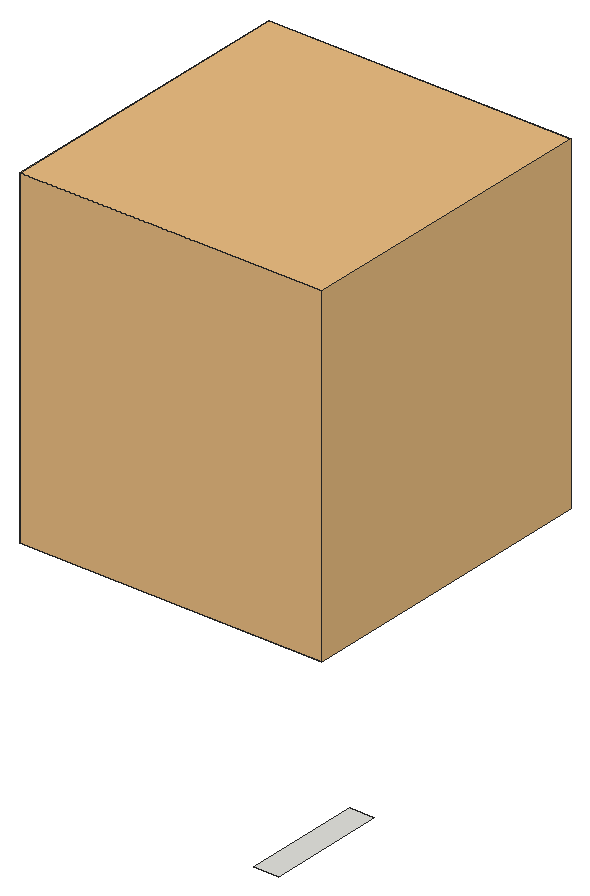
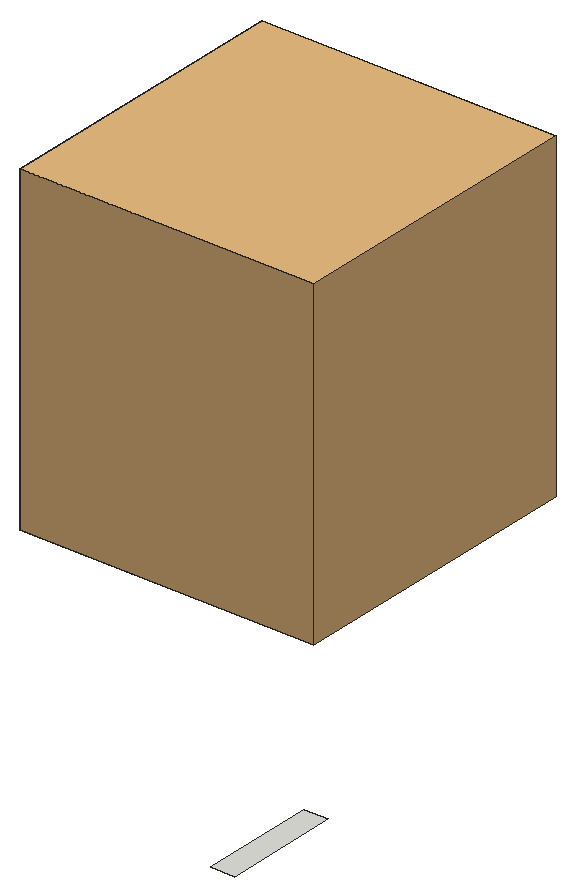
# SketchUp Ruby script. Lengths in inches.
U = 1.inch
M = Sketchup.active_model
def pt(a) = Geom::Point3d.new(a.map { |v| v * U })
def face(e, loops, mat)
  f = e.add_face(loops[0].map { |a| pt(a) })
  loops[1..].each { |l| e.add_face(l.map { |a| pt(a) }).erase! }
  f.material = f.back_material = mat if mat
  f
end
# faces: each face lists its corners as indices into pts; further lists are holes
def faces(e, pts, list, mat = nil) = list.each { |f| face(e, (f[0].is_a?(Array) ? f : [f]).map { |l| l.map { |i| pts[i] } }, mat) }
# xy, xz, yz: faces in a plane at the given z, y or x. An outline is a flat list of corners, or four numbers for a rectangle; further outlines are holes
def ring(l) = l.size == 4 ? [[l[0], l[1]], [l[2], l[1]], [l[2], l[3]], [l[0], l[3]]] : l.each_slice(2).to_a
def flat(e, list, mat, &to3) = list.each { |f| face(e, (f[0].is_a?(Array) ? f : [f]).map { |l| ring(l).map { |u, v| to3.(u, v) } }, mat) }
def xy(e, z, list, mat = nil) = flat(e, list, mat) { |x, y| [x, y, z] }
def xz(e, y, list, mat = nil) = flat(e, list, mat) { |x, z| [x, y, z] }
def yz(e, x, list, mat = nil) = flat(e, list, mat) { |y, z| [x, y, z] }
def lines(e, pts, list) = list.each { |a, b| e.add_line(pt(pts[a]), pt(pts[b])) }
# prism: a flat outline (further loops are holes) pulled along v
def prism(e, loops, v, mat = nil)
  f = face(e, loops, mat); d = Geom::Vector3d.new(v.map { |x| x * U })
  f.pushpull(f.normal.samedirection?(d) ? d.length : -d.length)
end
def box(e, o, s, mat = nil) = prism(e, [[o, [o[0] + s[0], o[1], o[2]], [o[0] + s[0], o[1] + s[1], o[2]], [o[0], o[1] + s[1], o[2]]]], [0, 0, s[2]], mat)
def at(x, y, z, deg = 0) = Geom::Transformation.translation(pt([x, y, z])) * Geom::Transformation.rotation(ORIGIN, Z_AXIS, deg.degrees)
def axes(o, x, y, z) = Geom::Transformation.new([*x, 0, *y, 0, *z, 0, *pt(o).to_a, 1])
def part(name) = M.definitions.add(name)
# library, detail: a bought-in or finely detailed component or shape, given as its bounding box
def library(name, o, s) = part(name).tap { |d| box(d.entities, o, s) }
def detail(e, o, s) = box(e.add_group.entities, o, s)
def put(e, d, t, mat = nil) = e.add_instance(d, t).tap { |i| i.material = mat if mat }
def group(e, t, mat = nil) = e.add_group.tap { |g| g.transformation = t; g.material = mat if mat }.entities
root = M.entities
c1 = library("chau cay",[-24.34,-109.24,0],[56.46,62.58,79.69])
xy(root,98.875,[[186.24,203.17,189.49,219.06]])
put(root,c1,axes([185.1,259.46,137.875],[0.71,0,0],[0,0.66,0],[0,0,0.5538]))
